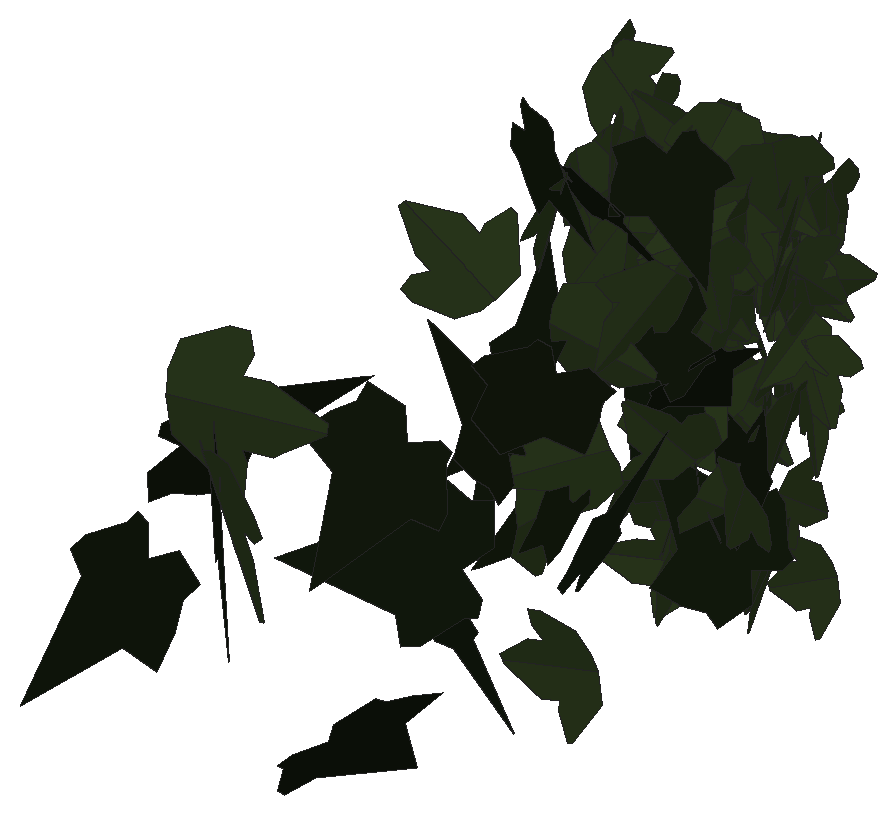
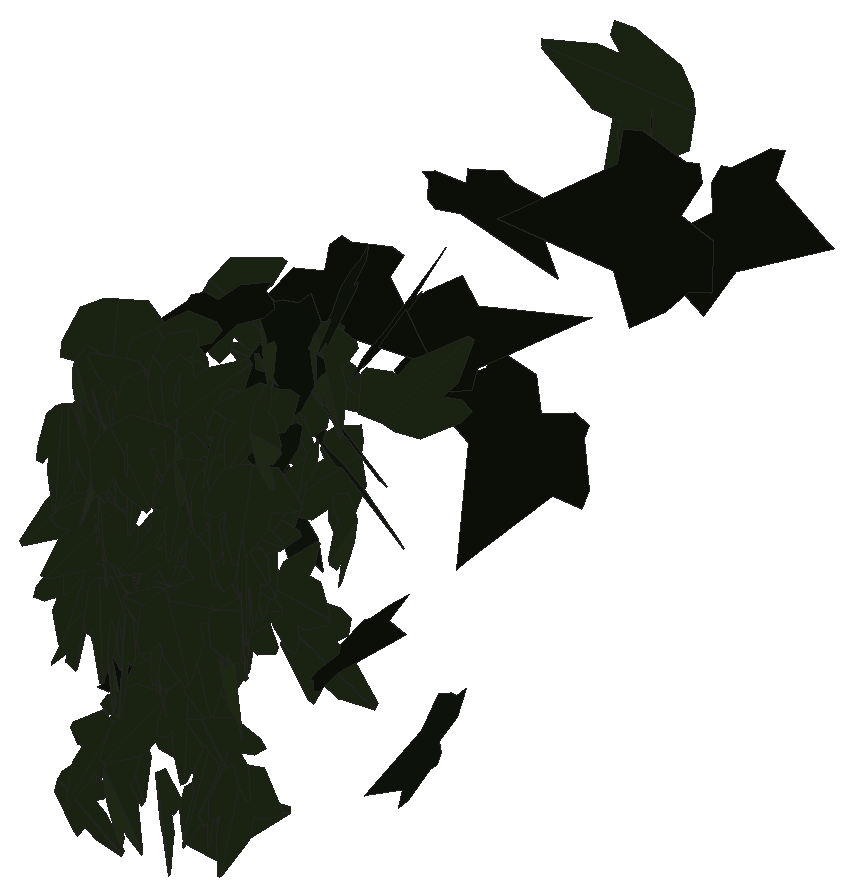
# SketchUp Ruby script. Lengths in inches.
U = 1.inch
M = Sketchup.active_model
def pt(a) = Geom::Point3d.new(a.map { |v| v * U })
def face(e, loops, mat)
  f = e.add_face(loops[0].map { |a| pt(a) })
  loops[1..].each { |l| e.add_face(l.map { |a| pt(a) }).erase! }
  f.material = f.back_material = mat if mat
  f
end
# faces: each face lists its corners as indices into pts; further lists are holes
def faces(e, pts, list, mat = nil) = list.each { |f| face(e, (f[0].is_a?(Array) ? f : [f]).map { |l| l.map { |i| pts[i] } }, mat) }
# xy, xz, yz: faces in a plane at the given z, y or x. An outline is a flat list of corners, or four numbers for a rectangle; further outlines are holes
def ring(l) = l.size == 4 ? [[l[0], l[1]], [l[2], l[1]], [l[2], l[3]], [l[0], l[3]]] : l.each_slice(2).to_a
def flat(e, list, mat, &to3) = list.each { |f| face(e, (f[0].is_a?(Array) ? f : [f]).map { |l| ring(l).map { |u, v| to3.(u, v) } }, mat) }
def xy(e, z, list, mat = nil) = flat(e, list, mat) { |x, y| [x, y, z] }
def xz(e, y, list, mat = nil) = flat(e, list, mat) { |x, z| [x, y, z] }
def yz(e, x, list, mat = nil) = flat(e, list, mat) { |y, z| [x, y, z] }
def lines(e, pts, list) = list.each { |a, b| e.add_line(pt(pts[a]), pt(pts[b])) }
# prism: a flat outline (further loops are holes) pulled along v
def prism(e, loops, v, mat = nil)
  f = face(e, loops, mat); d = Geom::Vector3d.new(v.map { |x| x * U })
  f.pushpull(f.normal.samedirection?(d) ? d.length : -d.length)
end
def box(e, o, s, mat = nil) = prism(e, [[o, [o[0] + s[0], o[1], o[2]], [o[0] + s[0], o[1] + s[1], o[2]], [o[0], o[1] + s[1], o[2]]]], [0, 0, s[2]], mat)
def at(x, y, z, deg = 0) = Geom::Transformation.translation(pt([x, y, z])) * Geom::Transformation.rotation(ORIGIN, Z_AXIS, deg.degrees)
def axes(o, x, y, z) = Geom::Transformation.new([*x, 0, *y, 0, *z, 0, *pt(o).to_a, 1])
def part(name) = M.definitions.add(name)
# library, detail: a bought-in or finely detailed component or shape, given as its bounding box
def library(name, o, s) = part(name).tap { |d| box(d.entities, o, s) }
def detail(e, o, s) = box(e.add_group.entities, o, s)
def put(e, d, t, mat = nil) = e.add_instance(d, t).tap { |i| i.material = mat if mat }
def group(e, t, mat = nil) = e.add_group.tap { |g| g.transformation = t; g.material = mat if mat }.entities
root = M.entities
M.materials.add("efeu1").color = [18, 25, 13]
M.materials.add("efeu2").color = [43, 57, 29]
c1 = part("ivyleaf_10")
p = [[0,0.5,-0.03],[-0.0625,2.02,-0.43],[-0.19,2.01,-0.46],[-0.54,1.05,-0.29],[-0.52,0.625,-0.18],[-0.83,0.76,-0.28],
  [-1.16,0.64,-0.33],[-1.15,0.33,-0.24],[-0.77,-0.39,0.02],[-0.3,-0.51,0.16],[0.04,-0.48,0.23],[-0.02,2.01,-0.4375],
  [-0.06,2.01,-0.43],[0.04,-0.49,0.23],[0.67,-0.49,0.14],[1.38,0.36,-0.2],[1.375,0.51,-0.24],[0.81,0.65,-0.19],
  [0.62,0.59,-0.15],[0.6,1.09,-0.28],[0.5,1.23,-0.31]]
faces(c1.entities,p,[[0,1,2,3,4,5,6,7,8,9,10],[11,12,0,13,14,15,16,17,18,19,20]],"efeu2")
c2 = part("ivyleaf_9")
p = [[1.54,2.16,1.25],[1.36,2.04,1.19],[-0.21,0.99,0.68],[-0.71,1.11,0.82],[-0.85,0.86,0.67],[-0.8,0.17,0.21],
  [-0.9,-0.01,0.1],[-0.67,-0.16,-0.02],[-0.08,-0.08,-0.05],[-0.03,-0.6,-0.4],[0.65,-0.88,-0.66],[0.83,-0.6,-0.49],
  [1.29,-0.42,-0.43],[1.8125,-0.07,-0.26],[1.21,0.44,0.15]]
faces(c2.entities,p,[[0,1,2,3,4,5,6,7,8,9,10,11,12,13,14]],"efeu1")
put(root,c1,axes([504.18,138.0625,172.01],[0.23642,-0.31715,0.55644],[0.33783,-0.44217,-0.39556],[0.54414,0.41232,0.00382]))
put(root,c1,axes([504.52,137.9,169.58],[0.14401,-0.58308,-0.26247],[-0.01773,0.26531,-0.59909],[0.63918,0.13873,0.04252]))
put(root,c2,axes([504.41,135.66,166.93],[-0.19114,-0.61525,0.418],[-0.10568,-0.40474,-0.64406],[0.73627,-0.21782,0.01607]))
put(root,c1,axes([504.59,137.82,170.86],[-0.3945,-0.48964,-0.10766],[0.07297,0.07946,-0.62875],[0.496,-0.40113,0.00687]))
put(root,c1,axes([504.51,136.65,170.63],[-0.09218,0.7292,-0.07445],[0.00803,-0.07403,-0.73501],[-0.73295,-0.09252,0.00131]))
put(root,c2,axes([504.16,133.59,164.46],[0.55443,-0.55314,0.02285],[0.02196,-0.0111,-0.7848],[0.59746,0.51371,0.00764]))
put(root,c1,axes([504.88,133.57,170.3],[0.34551,0.56535,0.47201],[-0.24836,-0.39133,0.67554],[0.74255,-0.39395,0.00632]))
put(root,c1,axes([504.8,137.67,168.79],[0.35723,-0.47449,-0.34447],[-0.1007,0.34772,-0.58341],[0.57764,0.35406,0.11132]))
put(root,c1,axes([504.8125,137.87,169.92],[-0.07381,-0.60581,0.323],[-0.02429,-0.32235,-0.61015],[0.68611,-0.07659,0.01315]))
put(root,c1,axes([504.62,137.3,172.11],[0.16699,0.56416,0.32934],[0.09088,0.31656,-0.58835],[-0.6469,0.19011,0.00236]))
put(root,c1,axes([504.9,137.58,169.69],[-0.20033,-0.65298,0.10318],[-0.02443,-0.10043,-0.683],[0.66063,-0.20172,0.00603]))
put(root,c1,axes([505.0625,138.08,165.27],[0.02473,0.12931,-0.63154],[-0.15639,0.61433,0.11967],[0.62539,0.14851,0.0549]))
put(root,c1,axes([504.9375,137.61,165.125],[-0.10115,-0.62725,-0.29772],[0.0837,0.28766,-0.63447],[0.68925,-0.12699,0.03335]))
put(root,c1,axes([504.98,137.87,170.17],[0.04042,-0.64841,-0.01327],[-0.00082,0.01325,-0.64967],[0.64854,0.04043,0]))
put(root,c1,axes([504.67,138.09,166.89],[0.10489,-0.29457,-0.5666],[0.26581,-0.50195,0.31016],[-0.58065,-0.28299,0.03964]))
put(root,c1,axes([505.11,138.27,165.65],[0.09905,-0.39957,-0.50565],[-0.02209,0.50918,-0.40669],[0.64409,0.07892,0.06381]))
put(root,c1,axes([505.53,137.4375,169.75],[0.02653,0.03215,-0.63523],[-0.63561,0.16771,-0.01544],[0.17989,0.58783,0.03914]))
put(root,c1,axes([505.21,138.02,170.71],[0.01564,-0.62675,0.13313],[0.02748,-0.13239,-0.6265],[0.64014,0.02099,0.02364]))
put(root,c1,axes([504.97,137.81,168.92],[0.4893,0.35894,-0.34003],[0.27767,0.19633,0.60681],[0.40909,-0.56257,-0.00518]))
put(root,c1,axes([505.18,137.625,168.25],[-0.03985,-0.25558,0.66849],[0.15208,-0.65726,-0.24222],[0.69934,0.12837,0.09077]))
put(root,c1,axes([505.33,137.86,166.09],[0.61472,0.12094,-0.20602],[-0.20375,-0.03154,-0.62645],[-0.12473,0.64756,0.00797]))
put(root,c1,axes([505.36,137.35,171.75],[0.05697,-0.54142,-0.35837],[0.1013,0.36275,-0.53194],[0.64133,-0.0092,0.11586]))
put(root,c2,axes([505.04,126.43,170.62],[0.08421,0.73326,-0.7434],[-0.00032,0.7169,0.76478],[1.10595,-0.05563,0.05683]))
put(root,c1,axes([505.46,138.33,170.88],[-0.11829,-0.58008,-0.2439],[0.08485,0.2312,-0.59104],[0.62353,-0.14151,0.03416]))
put(root,c1,axes([505.96,137.29,164.1],[-0.04167,-0.03002,-0.67662],[-0.62906,-0.24951,0.04981],[-0.251,0.63032,-0.01251]))
put(root,c1,axes([505.64,137.96,167.6875],[-0.23728,-0.60961,0.11718],[-0.0161,-0.11937,-0.65357],[0.62057,-0.23619,0.02785]))
put(root,c1,axes([505.47,135.74,167.63],[0.09869,-0.42814,0.5521],[0.17265,-0.52534,-0.43825],[0.67698,0.19639,0.03129]))
put(root,c1,axes([505.59,134.65,171.54],[0.18527,-0.65746,0.00686],[0.00936,-0.00455,-0.70661],[0.71003,0.17161,0.00752]))
put(root,c2,axes([505.36,134.29,172.61],[0.55018,-0.38638,-0.38017],[-0.30905,0.22757,-0.66491],[0.48423,0.58425,0.00757]))
put(root,c1,axes([505.66,138.09,171.04],[0.17723,-0.61623,-0.05313],[-0.01786,0.05015,-0.6412],[0.61826,0.1781,-0.0033]))
put(root,c1,axes([505.55,137.66,170.45],[-0.13522,-0.34351,-0.52703],[0.1905,0.4914,-0.36916],[0.59956,-0.2336,-0.00156]))
put(root,c1,axes([505.72,137.41,165.07],[0.33623,-0.54381,-0.17276],[-0.08317,0.15167,-0.6393],[0.5645,0.34625,0.00871]))
put(root,c2,axes([505.69,124.51,169.58],[-0.03314,-0.0077,-1.01183],[0.38592,-0.90546,-0.00427],[-0.97735,-0.35727,0.03262]))
put(root,c1,axes([505.71,137.96,166.58],[-0.13707,-0.61505,-0.13798],[0.03501,0.13356,-0.63012],[0.62936,-0.14138,0.005]))
put(root,c1,axes([505.84,138.26,168.35],[-0.25499,-0.57901,0.11083],[-0.03415,-0.10604,-0.63257],[0.58853,-0.25702,0.01131]))
put(root,c1,axes([505.51,136.2,171.63],[-0.05926,0.06737,-0.75086],[0.28307,-0.69608,-0.0848],[-0.69872,-0.28771,0.02933]))
put(root,c2,axes([506.08,133.48,169.32],[-0.60878,0.33475,-0.12706],[-0.12472,0.0447,0.68149],[0.36409,0.57504,0.02099]))
put(root,c1,axes([505.55,136.875,169.94],[-0.17251,-0.18034,-0.73188],[0.491,0.54278,-0.24947],[0.57191,-0.52038,-0.00658]))
put(root,c1,axes([505.89,137.11,171.02],[0.36678,-0.53806,-0.0015],[-0.00214,0.00036,-0.65118],[0.53806,0.36678,-0.00156]))
put(root,c1,axes([506.29,137.32,171.42],[-0.41244,-0.14407,-0.5147],[-0.49061,-0.1559,0.43677],[-0.21206,0.64087,-0.00946]))
put(root,c1,axes([505.875,138.25,169.82],[0.01271,-0.13437,-0.62764],[0.12297,0.61664,-0.12952],[0.62997,-0.11766,0.03795]))
put(root,c1,axes([506.07,135.96,169.25],[0.19398,-0.59324,-0.38705],[-0.12087,0.36769,-0.62415],[0.69795,0.22856,-0.00051]))
put(root,c2,axes([505.49,135.9375,169.93],[0.63259,-0.47981,0.03558],[0.02506,-0.02583,-0.79395],[0.48048,0.63306,-0.00543]))
put(root,c1,axes([505.79,133.82,167.91],[-0.349,0.40632,-0.35157],[0.21695,-0.27208,-0.53981],[-0.52801,-0.38036,0.01058]))
put(root,c1,axes([506.04,138.19,167.61],[0.13515,-0.61537,-0.1097],[-0.00123,0.11197,-0.62964],[0.62507,0.13328,0.02248]))
put(root,c1,axes([506.14,138.11,164.82],[0.25741,-0.54775,-0.2026],[-0.06259,0.19426,-0.60472],[0.58066,0.26376,0.02463]))
put(root,c1,axes([506.01,137.76,167.77],[0.07665,-0.44703,0.44825],[0.07738,0.45475,0.44028],[-0.62831,0.00148,0.10891]))
put(root,c1,axes([505.8,135.1,170.04],[0.61002,-0.24405,-0.38716],[0.36728,-0.1515,0.63991],[-0.3102,-0.6593,-0.00373]))
put(root,c1,axes([506.59,136.67,166.83],[0.49489,0.17402,0.59062],[-0.57493,-0.14063,0.52317],[0.22039,-0.75761,0.03855]))
put(root,c1,axes([506,137.43,169.6],[-0.05697,-0.16691,-0.61965],[0.24281,-0.58145,0.1343],[-0.59403,-0.22166,0.11432]))
put(root,c2,axes([505.82,134.91,171.63],[0.7335,-0.17788,0.07349],[0.0738,-0.018,-0.73016],[0.19309,0.68259,-0.0001]))
put(root,c1,axes([506.42,136.09,170.01],[0.10011,-0.48566,-0.46519],[-0.08425,0.44046,-0.51418],[0.70808,0.12107,0.00459]))
put(root,c1,axes([506.73,137.68,167.71],[-0.4351,-0.12941,0.50407],[-0.48783,-0.12743,-0.45379],[0.18126,-0.65357,-0.01133]))
put(root,c1,axes([506.19,138.32,166.4],[-0.47798,-0.15298,-0.33736],[0.3304,0.10785,-0.48699],[0.20214,-0.53802,-0.0017]))
put(root,c1,axes([506.48,136.45,168.77],[-0.08041,-0.13007,-0.65889],[-0.18033,-0.63505,0.14737],[-0.64694,0.19318,0.04081]))
put(root,c1,axes([506.49,135.63,166.8125],[-0.03787,-0.5861,-0.39692],[0.01155,0.39692,-0.58721],[0.70776,-0.03784,-0.01166]))
put(root,c1,axes([506.45,136.41,164.74],[0.16981,-0.51788,-0.43212],[0.08502,0.45848,-0.51607],[0.6691,0.07318,0.17524]))
put(root,c1,axes([506.79,137.39,167.1],[0.41957,-0.01566,0.52668],[-0.45096,0.35157,0.34443],[-0.30995,-0.53272,0.21183]))
put(root,c1,axes([506.62,136.74,171.59],[0.0662,-0.51706,-0.39918],[-0.0108,0.4003,-0.5203],[0.65313,0.05903,0.03186]))
put(root,c1,axes([506.43,136.61,169.25],[-0.41287,-0.30801,-0.48789],[0.37312,0.31507,-0.51466],[0.44009,-0.55608,-0.02137]))
put(root,c1,axes([506.67,137.26,165.97],[0.26341,-0.57839,0.06683],[0.02242,-0.06322,-0.63552],[0.58181,0.2643,-0.00577]))
put(root,c1,axes([506.65,136.99,168.8125],[-0.03041,0.37325,0.56313],[-0.0896,0.53562,-0.38848],[-0.70459,-0.08422,0.02509]))
put(root,c2,axes([506.13,125.6875,170.98],[-0.15346,0.0598,-1.08805],[1.08768,-0.28392,-0.15913],[-0.31271,-1.01691,-0.01955]))
put(root,c1,axes([506.79,138.39,171.08],[-0.20615,-0.5524,0.24581],[-0.03629,-0.24793,-0.58761],[0.60354,-0.2036,0.04863]))
put(root,c1,axes([507.08,136.37,165.93],[-0.47963,0.27362,0.57924],[-0.51466,0.2663,-0.55195],[-0.38147,-0.70331,0.01636]))
put(root,c1,axes([506.89,136.98,168.91],[-0.23845,-0.63166,0.16282],[-0.05621,-0.15281,-0.67517],[0.64988,-0.24499,0.00134]))
put(root,c1,axes([506.84,138.12,167.46],[0.35557,-0.39335,-0.35156],[-0.05951,0.39135,-0.49805],[0.52419,0.31124,0.18192]))
put(root,c1,axes([506.73,137.3,171.99],[0.0984,-0.57095,0.39731],[0.15184,-0.37396,-0.575],[0.67882,0.16641,0.07102]))
put(root,c1,axes([507.06,138.25,167.1],[0.07118,-0.16693,-0.61273],[-0.27758,0.54637,-0.1811],[0.57118,0.28632,-0.01165]))
put(root,c1,axes([506.97,137.14,171.46],[-0.54519,-0.39707,0.07042],[-0.06257,-0.03586,-0.6679],[0.4305,-0.50807,-0.00789]))
put(root,c1,axes([505.96,125.63,172.09],[0.06384,-0.02983,-1.10161],[1.12478,-0.19414,0.06613],[-0.21119,-1.04297,0.0192]))
put(root,c1,axes([506.81,137.01,169.31],[0.09866,-0.34057,0.59703],[0.17965,-0.56941,-0.3545],[0.66345,0.20483,0.00721]))
put(root,c1,axes([507.03,137.59,170.65],[0.12733,-0.57756,-0.38663],[-0.04549,0.3853,-0.59055],[0.69353,0.13131,0.03225]))
put(root,c1,axes([507,137.53,170.69],[-0.03218,-0.62457,0.24409],[0.02164,-0.24521,-0.62459],[0.67022,-0.02208,0.03188]))
put(root,c1,axes([507.5,132.71,164.81],[0.29913,-0.06878,-0.78147],[-0.73522,0.32246,-0.29166],[0.35148,0.73304,0.05498]))
put(root,c2,axes([506.74,135.81,168.56],[-0.04974,-0.72483,0.33388],[0.01213,-0.33518,-0.72584],[0.79794,-0.04009,0.03184]))
put(root,c1,axes([507.07,136.83,172.23],[0.42185,0.44066,-0.33269],[-0.25687,-0.21608,-0.61159],[-0.52903,0.4563,0.03167]))
put(root,c1,axes([507.29,136.53,170.72],[-0.21366,-0.03349,0.6352],[-0.2504,-0.58991,-0.11175],[0.61132,-0.25334,0.17624]))
put(root,c1,axes([507.14,138.05,164.57],[0.30335,-0.60504,0.24995],[0.10514,-0.22688,-0.67679],[0.64614,0.32098,-0.00722]))
put(root,c1,axes([506.99,124.77,171.37],[-0.78207,0.64745,-0.35919],[0.27017,-0.23835,-1.01017],[-0.74504,-0.76606,0.01072]))
put(root,c2,axes([507.45,131.07,169.36],[-0.06045,-0.72835,0.27471],[0.02034,0.26348,0.75972],[-0.8365,0.05904,-0.00138]))
put(root,c1,axes([507.46,136.98,171.22],[-0.22628,-0.60056,0.38096],[-0.12163,-0.36121,-0.64167],[0.70072,-0.25663,0.01164]))
put(root,c1,axes([507.36,138.1,167.9375],[0.06199,-0.60669,-0.21449],[-0.02542,0.21301,-0.60984],[0.64299,0.06691,-0.00343]))
put(root,c1,axes([507.44,136.5,165.32],[0.16537,0.25415,-0.49012],[-0.2675,-0.40094,-0.30857],[-0.51267,0.29118,0.00291]))
put(root,c1,axes([507.39,138.1,165.36],[-0.00343,0.31981,0.52332],[-0.18599,0.48126,-0.31924],[-0.61647,-0.14698,0.0934]))
put(root,c1,axes([507.25,132,167.72],[-0.02295,-0.06833,-0.85343],[0.24653,0.78822,-0.07441],[0.85447,-0.22925,-0.00145]))
put(root,c2,axes([507.1,135.48,172.3125],[-0.04843,-0.59192,-0.34956],[0.06945,0.33166,-0.61634],[0.73186,-0.07064,0.03536]))
put(root,c1,axes([507.39,137.22,171.08],[-0.48366,-0.30103,-0.13161],[0.11435,0.06934,-0.56118],[0.33362,-0.46017,0.00154]))
put(root,c1,axes([507.28,136.72,170.69],[-0.40445,-0.41868,-0.3173],[0.30957,0.14612,-0.57446],[0.46605,-0.4604,0.10622]))
put(root,c1,axes([506.8125,133.59,170.05],[-0.05505,0.03823,-0.87724],[0.81603,-0.32231,-0.06525],[-0.32421,-0.81774,-0.01529]))
put(root,c2,axes([507.93,132.14,168.47],[-0.79314,0.41514,-0.05086],[0.04523,-0.0253,-0.87735],[-0.44919,-0.73558,0.00147]))
put(root,c2,axes([508.06,129.1,168.36],[-0.41144,-0.15886,0.83802],[-0.80712,-0.30134,-0.42925],[0.36787,-0.83882,-0.0045]))
put(root,c1,axes([507.88,138.15,170.9375],[-0.40372,0.1312,0.47502],[-0.48271,0.01837,-0.41533],[-0.09923,-0.62313,0.08777]))
put(root,c1,axes([507.58,137.76,169.48],[0.21609,-0.56641,-0.23081],[-0.0365,0.23242,-0.60452],[0.61054,0.21437,0.04555]))
put(root,c2,axes([508,134.79,169.92],[-0.65584,-0.01468,0.28618],[-0.29711,-0.00625,-0.63173],[0.01723,-0.66666,-0.00038]))
put(root,c2,axes([508.02,136.2,166.35],[-0.11247,0.22175,0.77835],[-0.3362,0.70202,-0.24858],[-0.73618,-0.35447,-0.00539]))
put(root,c1,axes([507.61,137.27,165.08],[0.03032,-0.63755,0.09672],[-0.00355,-0.09699,-0.63822],[0.64484,0.02944,-0.00806]))
put(root,c1,axes([507.41,136.12,166.22],[-0.24381,-0.34169,-0.54236],[0.30795,0.44648,-0.41972],[0.5622,-0.39274,-0.0053]))
put(root,c1,axes([507.34,138.1,169.32],[-0.37761,-0.27584,-0.44025],[0.3955,0.20029,-0.46471],[0.33688,-0.54432,0.0521]))
put(root,c2,axes([508.04,136.2,165.26],[-0.60554,-0.54413,-0.08264],[-0.06118,-0.05556,0.8141],[-0.54696,0.60862,0.00043]))
put(root,c2,axes([507.57,126.77,166.18],[0.43258,0.83927,0.30399],[0.1118,0.27437,-0.96683],[-0.95327,0.41303,0.02455]))
put(root,c1,axes([507.71,137.72,170.24],[0.32092,-0.12287,-0.5951],[-0.13783,0.64074,-0.20662],[0.59182,0.21585,0.27458]))
put(root,c1,axes([507.96,138.09,164.19],[0.30784,-0.14818,-0.54839],[-0.49978,0.22584,-0.34158],[0.27002,0.58693,-0.00702]))
put(root,c2,axes([507.91,128.02,170.86],[-0.85074,-0.33306,-0.10211],[0.09731,0.03902,-0.88944],[0.36216,-0.79285,-0.00088]))
put(root,c1,axes([507.74,135.64,170.63],[-0.25331,-0.59351,-0.16687],[0.11457,0.13009,-0.66172],[0.65404,-0.25266,0.05128]))
put(root,c1,axes([507.35,137.2,171.37],[0.36061,0.18849,0.51579],[0.39426,0.34068,-0.40013],[-0.38228,0.52917,0.07388]))
put(root,c1,axes([507.68,137.44,170],[0.35514,0.54045,-0.06918],[-0.06101,-0.04343,-0.6574],[-0.58492,0.33267,0.02657]))
put(root,c1,axes([507.61,136.74,171],[0.03957,-0.18956,-0.54795],[0.08336,-0.52125,0.20061],[-0.59896,-0.08507,-0.00828]))
put(root,c1,axes([507.8125,137.92,168.56],[0.18062,0.31708,-0.45206],[-0.20039,-0.39328,-0.3726],[-0.54543,0.24949,-0.01281]))
put(root,c1,axes([507.88,137.56,169.98],[0.20603,-0.57003,-0.26053],[-0.04631,0.25965,-0.60473],[0.62503,0.20714,0.04108]))
put(root,c2,axes([508.11,131.4,170.66],[0.05623,0.20799,-0.77196],[-0.13851,-0.73126,-0.22245],[-0.82093,0.13763,-0.01535]))
put(root,c1,axes([507.93,137.36,167.5],[0.08532,-0.62946,0.06615],[0.00305,-0.06634,-0.63519],[0.63292,0.08517,-0.00585]))
put(root,c1,axes([508.44,131.875,169.24],[-0.32794,-0.09444,0.71857],[-0.61631,-0.3995,-0.31761],[0.43289,-0.64031,0.09218]))
put(root,c1,axes([507.87,137.98,168.07],[-0.47706,-0.36593,-0.12953],[0.20429,-0.0397,-0.57641],[0.36407,-0.45723,0.15371]))
put(root,c1,axes([507.99,137.77,171.55],[0.25327,-0.67703,0.0631],[0.02727,-0.05717,-0.72283],[0.67942,0.25467,0.00549]))
put(root,c1,axes([507.88,138.03,167.31],[-0.08151,0.53132,-0.15878],[0.02592,-0.1508,-0.55812],[-0.59649,-0.07915,-0.00255]))
put(root,c2,axes([507.95,132.41,166.91],[-0.3617,0.76048,-0.00181],[-0.02296,-0.00747,0.86388],[0.82099,0.33483,0.02337]))
put(root,c1,axes([508.07,138.22,170.91],[-0.02718,-0.6227,-0.19016],[0.05247,0.18761,-0.62186],[0.64897,-0.04125,0.04231]))
put(root,c2,axes([508.1,134.6875,169.2],[0.25426,0.61361,0.13842],[0.04456,0.12672,-0.68348],[-0.67665,0.23891,0.00701]))
put(root,c1,axes([508.14,136.8,172.13],[-0.51842,-0.54364,-0.07649],[0.05202,0.05609,-0.7512],[0.54652,-0.52102,-0.00106]))
put(root,c1,axes([508.01,137.41,169.875],[-0.234,-0.42443,-0.45458],[0.20481,0.40601,-0.48451],[0.58723,-0.31073,-0.01216]))
put(root,c1,axes([508.04,137.29,170.9375],[0.37657,-0.5015,0.19223],[0.11104,-0.157,-0.62712],[0.52548,0.39256,-0.00524]))
put(root,c1,axes([508.3,133.75,171.22],[-0.13647,-0.56033,0.49559],[-0.10549,-0.46645,-0.59735],[0.78738,-0.15961,0.00587]))
put(root,c1,axes([508.02,137.69,169.64],[-0.11649,-0.28765,-0.66456],[0.25292,0.61455,-0.31034],[0.67854,-0.27846,0.00158]))
put(root,c1,axes([508.42,134.18,168.28],[-0.45178,-0.29224,-0.46535],[-0.34236,-0.32178,0.52678],[-0.46468,0.5212,0.06431]))
put(root,c1,axes([508.48,135.63,166.85],[-0.5346,0.19435,0.3389],[-0.35963,0.03425,-0.5473],[-0.19643,-0.59165,0.07964]))
